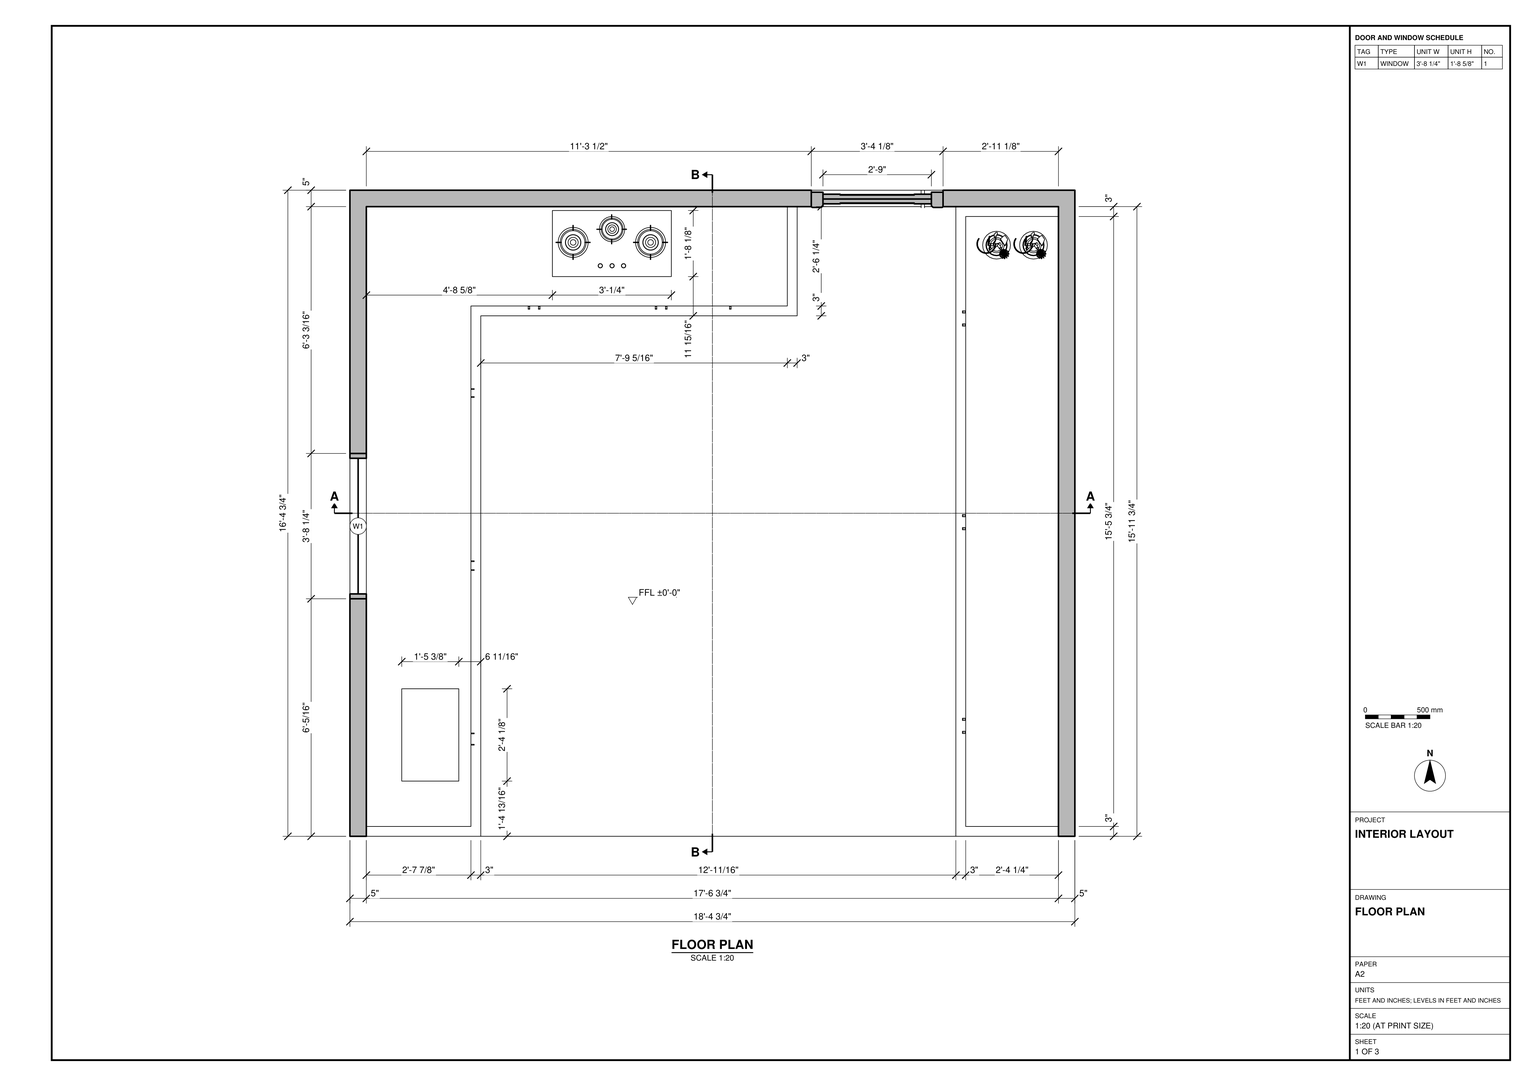
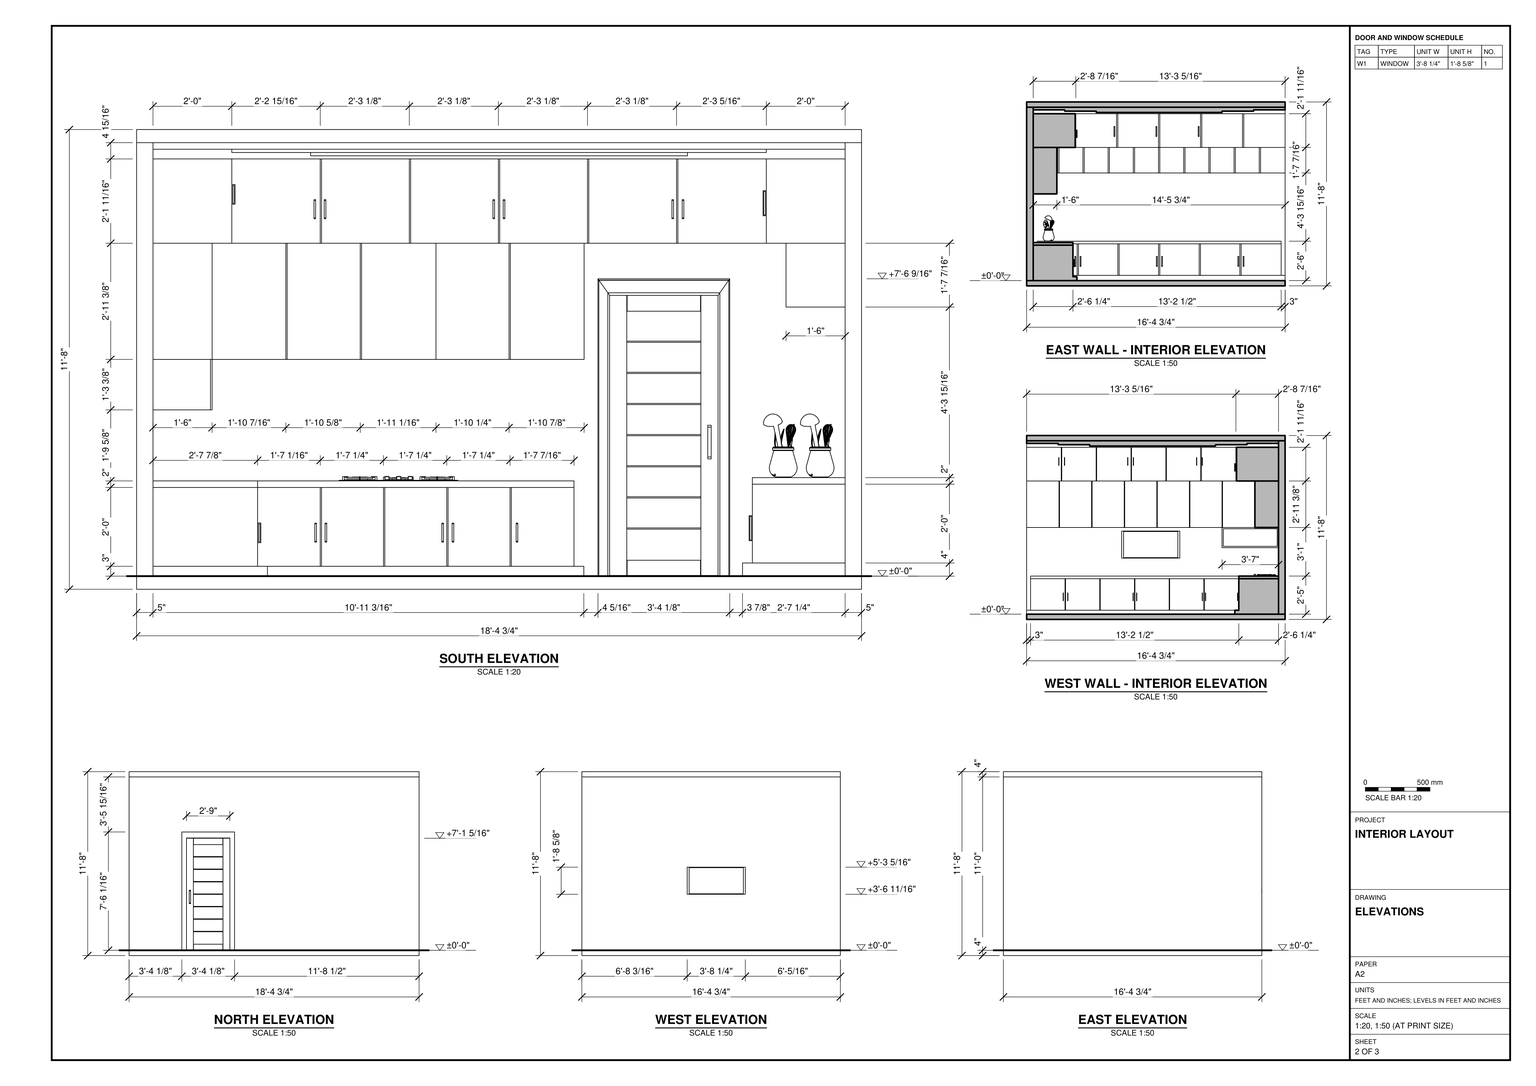
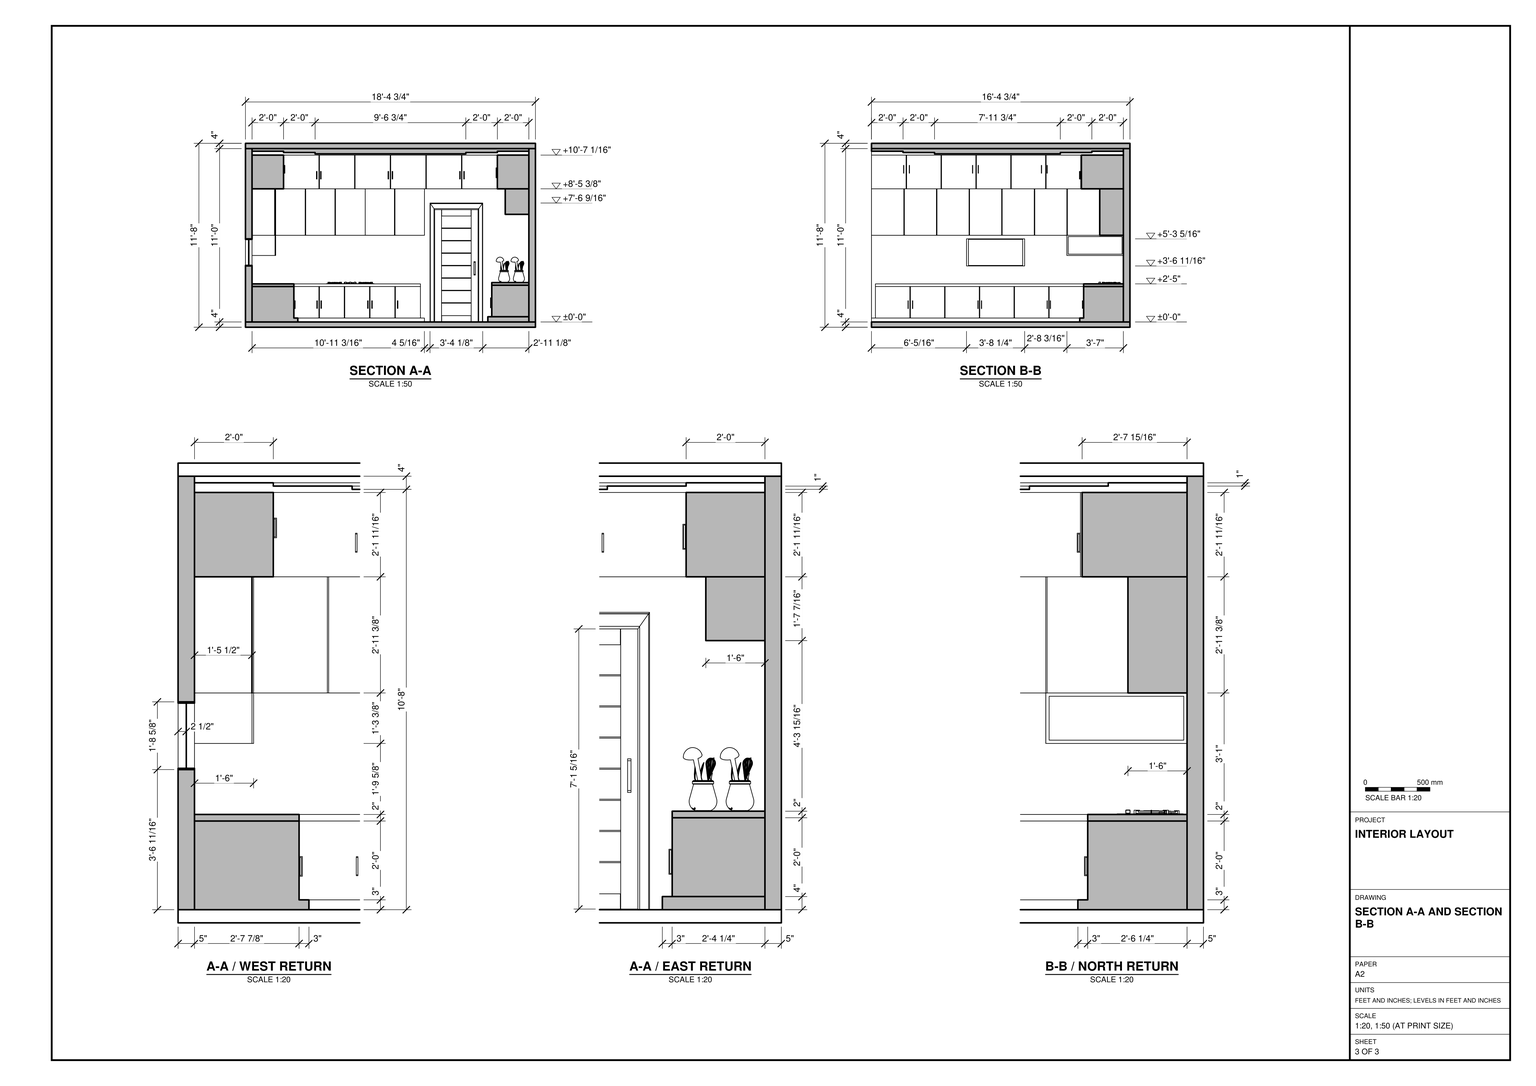
Build the kitchen in SketchUp using the plan, elevations and sections in task_files/diagram_01.pdf. Work in feet and inches. Set the finished floor at ±0'-0". The overall shell is 18'-4 3/4" wide from east to west, 16'-4 3/4" deep from north to south and 11'-8" high. Model the 5" walls on the north, east and west sides, leaving the south side open as drawn. Include the floor and ceiling slabs and the stepped ceiling detail shown in section.

Fit the framed window above the west worktop and the horizontally panelled door in the north wall. Run the west base cabinets around the northwest corner to form the cooktop counter, stopping short of the door. Include the rectangular inset near the open end of the west worktop. Place the separate straight cabinet run against the east wall. Use the return sections to set the counter depths, plinths and worktop thicknesses. Match the cabinet front divisions, handles and tiers of overhead storage to the elevations, including the cabinet row above the door.

Decor and loose items, including the cooktop and countertop utensil holders, may be any suitable library components. Keep shell elements and individual furniture or joinery pieces in separate groups or components, and use components for repeated parts. Save one SketchUp model as output_files/kitchen_interior_and_its_fitted_cabinetry.skp.

# SketchUp Ruby script. Lengths in inches.
U = 1.inch
M = Sketchup.active_model
def pt(a) = Geom::Point3d.new(a.map { |v| v * U })
def face(e, loops, mat)
  f = e.add_face(loops[0].map { |a| pt(a) })
  loops[1..].each { |l| e.add_face(l.map { |a| pt(a) }).erase! }
  f.material = f.back_material = mat if mat
  f
end
# faces: each face lists its corners as indices into pts; further lists are holes
def faces(e, pts, list, mat = nil) = list.each { |f| face(e, (f[0].is_a?(Array) ? f : [f]).map { |l| l.map { |i| pts[i] } }, mat) }
# xy, xz, yz: faces in a plane at the given z, y or x. An outline is a flat list of corners, or four numbers for a rectangle; further outlines are holes
def ring(l) = l.size == 4 ? [[l[0], l[1]], [l[2], l[1]], [l[2], l[3]], [l[0], l[3]]] : l.each_slice(2).to_a
def flat(e, list, mat, &to3) = list.each { |f| face(e, (f[0].is_a?(Array) ? f : [f]).map { |l| ring(l).map { |u, v| to3.(u, v) } }, mat) }
def xy(e, z, list, mat = nil) = flat(e, list, mat) { |x, y| [x, y, z] }
def xz(e, y, list, mat = nil) = flat(e, list, mat) { |x, z| [x, y, z] }
def yz(e, x, list, mat = nil) = flat(e, list, mat) { |y, z| [x, y, z] }
def lines(e, pts, list) = list.each { |a, b| e.add_line(pt(pts[a]), pt(pts[b])) }
# prism: a flat outline (further loops are holes) pulled along v
def prism(e, loops, v, mat = nil)
  f = face(e, loops, mat); d = Geom::Vector3d.new(v.map { |x| x * U })
  f.pushpull(f.normal.samedirection?(d) ? d.length : -d.length)
end
def box(e, o, s, mat = nil) = prism(e, [[o, [o[0] + s[0], o[1], o[2]], [o[0] + s[0], o[1] + s[1], o[2]], [o[0], o[1] + s[1], o[2]]]], [0, 0, s[2]], mat)
def at(x, y, z, deg = 0) = Geom::Transformation.translation(pt([x, y, z])) * Geom::Transformation.rotation(ORIGIN, Z_AXIS, deg.degrees)
def axes(o, x, y, z) = Geom::Transformation.new([*x, 0, *y, 0, *z, 0, *pt(o).to_a, 1])
def part(name) = M.definitions.add(name)
# library, detail: a bought-in or finely detailed component or shape, given as its bounding box
def library(name, o, s) = part(name).tap { |d| box(d.entities, o, s) }
def detail(e, o, s) = box(e.add_group.entities, o, s)
def put(e, d, t, mat = nil) = e.add_instance(d, t).tap { |i| i.material = mat if mat }
def group(e, t, mat = nil) = e.add_group.tap { |g| g.transformation = t; g.material = mat if mat }.entities
root = M.entities
M.materials.add("CROMO PERFIL METALICO").color = [144, 144, 144]
M.materials.add("Emissive").color = [255, 255, 255]
M.materials.add("MADEIRAS PORTAS MOD 4").color = [48, 37, 30]
M.materials.add("[Aluminum]").color = [179, 179, 179]
M.materials.add("[Carrera Marble]").color = [255, 255, 255]
M.materials.add("[Color D01]").color = [255, 242, 204]
M.materials.add("[Color E01]").color = [255, 255, 204]
M.materials.add("[Color F02]").color = [204, 255, 153]
M.materials.add("[Color M07]").color = [58, 58, 58]
M.materials.add("[Terrazzo Tile Accent]").color = [224, 221, 217]
M.materials.add("[Translucent Glass Gray]3").color = [128, 128, 128]
M.materials["[Translucent Glass Gray]3"].alpha = 0.3
M.materials.add("[Translucent Glass Sky Reflection]").color = [126, 138, 183]
M.materials["[Translucent Glass Sky Reflection]"].alpha = 0.52
M.materials.add("[Wood Cherry Original]").color = [152, 86, 42]
c1 = part("Group\#12")
xy(c1.entities,0,[[-0.79,16.82,0.71,16.85],[-0.79,16.85,0.71,23.5],[-0.79,23.5,0.71,23.53]],"CROMO PERFIL METALICO")
xy(c1.entities,0.39,[[-0.79,17.125,0.71,23.23]],"CROMO PERFIL METALICO")
xy(c1.entities,1.97,[[-0.79,16.73,0.71,17.125],[-0.79,23.23,0.71,23.62]],"CROMO PERFIL METALICO")
xz(c1.entities,16.73,[[-0.79,0.12,0.71,1.97]],"CROMO PERFIL METALICO")
xz(c1.entities,17.125,[[-0.79,0.39,0.71,1.97]],"CROMO PERFIL METALICO")
xz(c1.entities,23.23,[[-0.79,0.39,0.71,1.97]],"CROMO PERFIL METALICO")
xz(c1.entities,23.62,[[-0.79,0.09,0.71,0.12],[-0.79,0.12,0.71,1.97]],"CROMO PERFIL METALICO")
yz(c1.entities,-0.79,[[16.82,0,16.79,0.02,16.77,0.03,16.75,0.06,16.73,0.12,16.73,1.97,17.125,1.97,17.125,0.39,23.23,0.39,23.23,1.97,23.62,1.97,23.62,0.09,23.61,0.06,23.59,0.03,23.5625,0.02,23.53,0]],"CROMO PERFIL METALICO")
yz(c1.entities,0.71,[[16.82,0,23.53,0,23.5625,0.02,23.59,0.03,23.61,0.06,23.62,0.09,23.62,1.97,23.23,1.97,23.23,0.39,17.125,0.39,17.125,1.97,16.73,1.97,16.73,0.12,16.75,0.06,16.77,0.03,16.79,0.02]],"CROMO PERFIL METALICO")
p = [[-0.79,16.75,0.06],[-0.79,16.77,0.03],[0.71,16.77,0.03],[0.71,16.75,0.06],[-0.79,16.79,0.02],[0.71,16.79,0.02],
  [-0.79,16.82,0],[0.71,16.82,0],[-0.79,23.53,0],[-0.79,23.5625,0.02],[0.71,23.5625,0.02],[0.71,23.53,0],
  [-0.79,23.59,0.03],[0.71,23.59,0.03],[-0.79,23.61,0.06],[0.71,23.61,0.06],[-0.79,16.73,0.12],[-0.79,16.74,0.09],
  [0.71,16.74,0.09],[0.71,16.73,0.12],[-0.79,23.62,0.09],[0.71,23.62,0.09]]
faces(c1.entities,p,[[0,1,2,3],[1,4,5,2],[4,6,7,5],[8,9,10,11],[9,12,13,10],[12,14,15,13],[16,17,18,19],[17,0,3,18],
  [14,20,21,15]],"CROMO PERFIL METALICO")
c2 = part("Framed door panel")
xy(c2.entities,0.21,[[0,0,2.36,0,2.36,7.48,2.17,7.48,2.17,7.64,2.36,7.64,2.36,39.61,2.17,39.61,2.17,39.76,2.36,39.76,2.36,47.24,0,47.24]],"MADEIRAS PORTAS MOD 4")
xy(c2.entities,5.12,[[1.97,7.48,2.17,7.48,2.17,7.64,2.36,7.64,2.36,39.61,2.17,39.61,2.17,39.76,1.97,39.76]],"MADEIRAS PORTAS MOD 4")
xy(c2.entities,15.16,[[1.57,7.48,1.97,39.76]],"MADEIRAS PORTAS MOD 4")
xy(c2.entities,15.55,[[1.57,7.48,1.97,39.76]],"MADEIRAS PORTAS MOD 4")
xy(c2.entities,25.2,[[1.57,7.48,1.97,39.76]],"MADEIRAS PORTAS MOD 4")
xy(c2.entities,25.59,[[1.57,7.48,1.97,39.76]],"MADEIRAS PORTAS MOD 4")
xy(c2.entities,35.24,[[1.57,7.48,1.97,39.76]],"MADEIRAS PORTAS MOD 4")
xy(c2.entities,35.63,[[1.57,7.48,1.97,39.76]],"MADEIRAS PORTAS MOD 4")
xy(c2.entities,45.28,[[1.57,7.48,1.97,39.76]],"MADEIRAS PORTAS MOD 4")
xy(c2.entities,45.67,[[1.57,7.48,1.97,39.76]],"MADEIRAS PORTAS MOD 4")
xy(c2.entities,55.31,[[1.57,7.48,1.97,39.76]],"MADEIRAS PORTAS MOD 4")
xy(c2.entities,55.71,[[1.57,7.48,1.97,39.76]],"MADEIRAS PORTAS MOD 4")
xy(c2.entities,65.35,[[1.57,7.48,1.97,39.76]],"MADEIRAS PORTAS MOD 4")
xy(c2.entities,65.75,[[1.57,7.48,1.97,39.76]],"MADEIRAS PORTAS MOD 4")
xy(c2.entities,75.39,[[1.57,7.48,1.97,39.76]],"MADEIRAS PORTAS MOD 4")
xy(c2.entities,75.79,[[1.57,7.48,1.97,39.76]],"MADEIRAS PORTAS MOD 4")
xy(c2.entities,85.43,[[1.97,7.48,1.97,39.76,2.17,39.76,2.17,39.61,2.36,39.61,2.36,7.64,2.17,7.64,2.17,7.48]],"MADEIRAS PORTAS MOD 4")
xy(c2.entities,90.55,[[0,0,2.36,0,2.36,7.48,2.17,7.48,2.17,7.64,2.36,7.64,2.36,39.61,2.17,39.61,2.17,39.76,2.36,39.76,2.36,47.24,0,47.24]],"MADEIRAS PORTAS MOD 4")
xz(c2.entities,0,[[0,0.21,2.36,90.55]],"MADEIRAS PORTAS MOD 4")
xz(c2.entities,7.48,[[2.17,0.21,2.36,5.12],[1.97,5.12,2.36,15.16],[1.57,15.16,1.57,15.55,1.97,15.55,1.97,25.2,2.36,25.2,2.36,15.16],[1.57,25.2,1.57,25.59,1.97,25.59,1.97,35.24,2.36,35.24,2.36,25.2],[1.57,35.24,1.57,35.63,1.97,35.63,1.97,45.28,2.36,45.28,2.36,35.24],
  [1.57,45.28,1.57,45.67,1.97,45.67,1.97,55.31,2.36,55.31,2.36,45.28],[1.57,55.31,1.57,55.71,1.97,55.71,1.97,65.35,2.36,65.35,2.36,55.31],[1.57,65.35,1.57,65.75,1.97,65.75,1.97,75.39,2.36,75.39,2.36,65.35],[1.57,75.39,1.57,75.79,1.97,75.79,1.97,85.43,2.36,85.43,2.36,75.39],[2.17,85.43,2.36,90.55]],"MADEIRAS PORTAS MOD 4")
xz(c2.entities,7.64,[[2.17,0.21,2.36,5.12],[2.17,85.43,2.36,90.55]],"MADEIRAS PORTAS MOD 4")
xz(c2.entities,39.61,[[2.17,0.21,2.36,5.12],[2.17,85.43,2.36,90.55]],"MADEIRAS PORTAS MOD 4")
xz(c2.entities,39.76,[[2.17,0.21,2.36,5.12],[1.97,5.12,2.36,15.16],[1.57,15.16,2.36,15.16,2.36,25.2,1.97,25.2,1.97,15.55,1.57,15.55],[1.57,25.2,2.36,25.2,2.36,35.24,1.97,35.24,1.97,25.59,1.57,25.59],[1.57,35.24,2.36,35.24,2.36,45.28,1.97,45.28,1.97,35.63,1.57,35.63],
  [1.57,45.28,2.36,45.28,2.36,55.31,1.97,55.31,1.97,45.67,1.57,45.67],[1.57,55.31,2.36,55.31,2.36,65.35,1.97,65.35,1.97,55.71,1.57,55.71],[1.57,65.35,2.36,65.35,2.36,75.39,1.97,75.39,1.97,65.75,1.57,65.75],[1.57,75.39,2.36,75.39,2.36,85.43,1.97,85.43,1.97,75.79,1.57,75.79],[2.17,85.43,2.36,90.55]],"MADEIRAS PORTAS MOD 4")
xz(c2.entities,47.24,[[0,0.21,2.36,90.55]],"MADEIRAS PORTAS MOD 4")
yz(c2.entities,0,[[0,0.21,47.24,90.55]],"MADEIRAS PORTAS MOD 4")
yz(c2.entities,1.57,[[7.48,15.16,39.76,15.55],[7.48,25.2,39.76,25.59],[7.48,35.24,39.76,35.63],[7.48,45.28,39.76,45.67],[7.48,55.31,39.76,55.71],
  [7.48,65.35,39.76,65.75],[7.48,75.39,39.76,75.79]],"MADEIRAS PORTAS MOD 4")
yz(c2.entities,1.97,[[7.48,5.12,39.76,15.16],[7.48,15.55,39.76,25.2],[7.48,25.59,39.76,35.24],[7.48,35.63,39.76,45.28],[7.48,45.67,39.76,55.31],
  [7.48,55.71,39.76,65.35],[7.48,65.75,39.76,75.39],[7.48,75.79,39.76,85.43]],"MADEIRAS PORTAS MOD 4")
yz(c2.entities,2.17,[[7.48,0.21,7.64,5.12],[39.61,0.21,39.76,5.12],[7.48,85.43,7.64,90.55],[39.61,85.43,39.76,90.55]],"MADEIRAS PORTAS MOD 4")
yz(c2.entities,2.36,[[0,0.21,7.48,90.55],[7.64,0.21,39.61,5.12],[39.76,0.21,47.24,90.55],[7.64,85.43,39.61,90.55]],"MADEIRAS PORTAS MOD 4")
put(c2.entities,c1,axes([4.33,43.46,11.46],[0,-1,0],[0,0,1.575],[-1,0,0]))
c3 = part("Framed door panel \#1")
xy(c3.entities,0.21,[[0,0,2.36,0,2.36,7.48,2.17,7.48,2.17,7.64,2.36,7.64,2.36,39.61,2.17,39.61,2.17,39.76,2.36,39.76,2.36,47.24,0,47.24]],"MADEIRAS PORTAS MOD 4")
xy(c3.entities,5.12,[[1.97,7.48,2.17,7.48,2.17,7.64,2.36,7.64,2.36,39.61,2.17,39.61,2.17,39.76,1.97,39.76]],"MADEIRAS PORTAS MOD 4")
xy(c3.entities,15.16,[[1.57,7.48,1.97,39.76]],"MADEIRAS PORTAS MOD 4")
xy(c3.entities,15.55,[[1.57,7.48,1.97,39.76]],"MADEIRAS PORTAS MOD 4")
xy(c3.entities,25.2,[[1.57,7.48,1.97,39.76]],"MADEIRAS PORTAS MOD 4")
xy(c3.entities,25.59,[[1.57,7.48,1.97,39.76]],"MADEIRAS PORTAS MOD 4")
xy(c3.entities,35.24,[[1.57,7.48,1.97,39.76]],"MADEIRAS PORTAS MOD 4")
xy(c3.entities,35.63,[[1.57,7.48,1.97,39.76]],"MADEIRAS PORTAS MOD 4")
xy(c3.entities,45.28,[[1.57,7.48,1.97,39.76]],"MADEIRAS PORTAS MOD 4")
xy(c3.entities,45.67,[[1.57,7.48,1.97,39.76]],"MADEIRAS PORTAS MOD 4")
xy(c3.entities,55.31,[[1.57,7.48,1.97,39.76]],"MADEIRAS PORTAS MOD 4")
xy(c3.entities,55.71,[[1.57,7.48,1.97,39.76]],"MADEIRAS PORTAS MOD 4")
xy(c3.entities,65.35,[[1.57,7.48,1.97,39.76]],"MADEIRAS PORTAS MOD 4")
xy(c3.entities,65.75,[[1.57,7.48,1.97,39.76]],"MADEIRAS PORTAS MOD 4")
xy(c3.entities,75.39,[[1.57,7.48,1.97,39.76]],"MADEIRAS PORTAS MOD 4")
xy(c3.entities,75.79,[[1.57,7.48,1.97,39.76]],"MADEIRAS PORTAS MOD 4")
xy(c3.entities,85.43,[[1.97,7.48,1.97,39.76,2.17,39.76,2.17,39.61,2.36,39.61,2.36,7.64,2.17,7.64,2.17,7.48]],"MADEIRAS PORTAS MOD 4")
xy(c3.entities,90.55,[[0,0,2.36,0,2.36,7.48,2.17,7.48,2.17,7.64,2.36,7.64,2.36,39.61,2.17,39.61,2.17,39.76,2.36,39.76,2.36,47.24,0,47.24]],"MADEIRAS PORTAS MOD 4")
xz(c3.entities,0,[[0,0.21,2.36,90.55]],"MADEIRAS PORTAS MOD 4")
xz(c3.entities,7.48,[[2.17,0.21,2.36,5.12],[1.97,5.12,2.36,15.16],[1.57,15.16,1.57,15.55,1.97,15.55,1.97,25.2,2.36,25.2,2.36,15.16],[1.57,25.2,1.57,25.59,1.97,25.59,1.97,35.24,2.36,35.24,2.36,25.2],[1.57,35.24,1.57,35.63,1.97,35.63,1.97,45.28,2.36,45.28,2.36,35.24],
  [1.57,45.28,1.57,45.67,1.97,45.67,1.97,55.31,2.36,55.31,2.36,45.28],[1.57,55.31,1.57,55.71,1.97,55.71,1.97,65.35,2.36,65.35,2.36,55.31],[1.57,65.35,1.57,65.75,1.97,65.75,1.97,75.39,2.36,75.39,2.36,65.35],[1.57,75.39,1.57,75.79,1.97,75.79,1.97,85.43,2.36,85.43,2.36,75.39],[2.17,85.43,2.36,90.55]],"MADEIRAS PORTAS MOD 4")
xz(c3.entities,7.64,[[2.17,0.21,2.36,5.12],[2.17,85.43,2.36,90.55]],"MADEIRAS PORTAS MOD 4")
xz(c3.entities,39.61,[[2.17,0.21,2.36,5.12],[2.17,85.43,2.36,90.55]],"MADEIRAS PORTAS MOD 4")
xz(c3.entities,39.76,[[2.17,0.21,2.36,5.12],[1.97,5.12,2.36,15.16],[1.57,15.16,2.36,15.16,2.36,25.2,1.97,25.2,1.97,15.55,1.57,15.55],[1.57,25.2,2.36,25.2,2.36,35.24,1.97,35.24,1.97,25.59,1.57,25.59],[1.57,35.24,2.36,35.24,2.36,45.28,1.97,45.28,1.97,35.63,1.57,35.63],
  [1.57,45.28,2.36,45.28,2.36,55.31,1.97,55.31,1.97,45.67,1.57,45.67],[1.57,55.31,2.36,55.31,2.36,65.35,1.97,65.35,1.97,55.71,1.57,55.71],[1.57,65.35,2.36,65.35,2.36,75.39,1.97,75.39,1.97,65.75,1.57,65.75],[1.57,75.39,2.36,75.39,2.36,85.43,1.97,85.43,1.97,75.79,1.57,75.79],[2.17,85.43,2.36,90.55]],"MADEIRAS PORTAS MOD 4")
xz(c3.entities,47.24,[[0,0.21,2.36,90.55]],"MADEIRAS PORTAS MOD 4")
yz(c3.entities,0,[[0,0.21,47.24,90.55]],"MADEIRAS PORTAS MOD 4")
yz(c3.entities,1.57,[[7.48,15.16,39.76,15.55],[7.48,25.2,39.76,25.59],[7.48,35.24,39.76,35.63],[7.48,45.28,39.76,45.67],[7.48,55.31,39.76,55.71],
  [7.48,65.35,39.76,65.75],[7.48,75.39,39.76,75.79]],"MADEIRAS PORTAS MOD 4")
yz(c3.entities,1.97,[[7.48,5.12,39.76,15.16],[7.48,15.55,39.76,25.2],[7.48,25.59,39.76,35.24],[7.48,35.63,39.76,45.28],[7.48,45.67,39.76,55.31],
  [7.48,55.71,39.76,65.35],[7.48,65.75,39.76,75.39],[7.48,75.79,39.76,85.43]],"MADEIRAS PORTAS MOD 4")
yz(c3.entities,2.17,[[7.48,0.21,7.64,5.12],[39.61,0.21,39.76,5.12],[7.48,85.43,7.64,90.55],[39.61,85.43,39.76,90.55]],"MADEIRAS PORTAS MOD 4")
yz(c3.entities,2.36,[[0,0.21,7.48,90.55],[7.64,0.21,39.61,5.12],[39.76,0.21,47.24,90.55],[7.64,85.43,39.61,90.55]],"MADEIRAS PORTAS MOD 4")
put(c3.entities,c1,axes([4.33,3.7,11.46],[0,-1,0],[0,0,1.575],[-1,0,0]))
c4 = part("Agrupar\#1")
xy(c4.entities,0,[[-0.94,0,-1.34,0.39,-1.34,7.48,3.78,7.48,3.78,0.79,2.99,0],[52.125,0,51.34,0.79,51.34,7.48,56.46,7.48,56.46,0.39,56.0625,0]],"MADEIRAS PORTAS MOD 4")
xy(c4.entities,86.77,[[3.78,0.79,51.34,7.09],[3.78,7.09,51.34,7.48]],"MADEIRAS PORTAS MOD 4")
xy(c4.entities,91.89,[[-1.34,0.39,56.46,7.48]],"MADEIRAS PORTAS MOD 4")
xz(c4.entities,0,[[-0.94,0,2.99,0,2.99,87.56,-0.94,91.5],[52.125,0,56.0625,0,56.0625,91.5,52.125,87.56],[2.99,87.56,52.125,87.56,56.0625,91.5,-0.94,91.5]],"MADEIRAS PORTAS MOD 4")
xz(c4.entities,7.48,[[-1.34,0,3.78,0,3.78,86.77,51.34,86.77,51.34,0,56.46,0,56.46,91.89,-1.34,91.89]],"MADEIRAS PORTAS MOD 4")
yz(c4.entities,-1.34,[[0.39,0,7.48,91.89]],"MADEIRAS PORTAS MOD 4")
yz(c4.entities,3.78,[[0.79,0,7.48,86.77]],"MADEIRAS PORTAS MOD 4")
yz(c4.entities,51.34,[[0.79,0,7.09,86.77],[7.09,0,7.48,86.77]],"MADEIRAS PORTAS MOD 4")
yz(c4.entities,56.46,[[0.39,0,7.48,91.89]],"MADEIRAS PORTAS MOD 4")
p = [[-1.34,0.39,0],[-0.94,0,0],[-0.94,0,91.5],[-1.34,0.39,91.89],[3.78,0.79,86.77],[2.99,0,87.56],
  [2.99,0,0],[3.78,0.79,0],[51.34,0.79,0],[52.125,0,0],[52.125,0,87.56],[51.34,0.79,86.77],
  [56.46,0.39,91.89],[56.0625,0,91.5],[56.0625,0,0],[56.46,0.39,0]]
faces(c4.entities,p,[[0,1,2,3],[4,5,6,7],[8,9,10,11],[12,13,14,15],[11,10,5,4],[3,2,13,12]],"MADEIRAS PORTAS MOD 4")
c5 = part("建立群組\#94")
put(c5.entities,c2,axes([2.85,32.65,-0.17],[-0.65909,0,0],[0,-0.62402,0],[0,0,0.82113]),"MADEIRAS PORTAS MOD 4")
put(c5.entities,c3,axes([2.85,3.17,0],[0.65909,0,0],[0,0.62402,0],[0,0,0.82113]),"MADEIRAS PORTAS MOD 4")
put(c5.entities,c4,axes([5.58,0.83,0],[0,0.61989,0],[-0.65909,0,0],[0,0,0.8569]),"MADEIRAS PORTAS MOD 4")
c6 = part("元件\#5")
put(c6.entities,c5,axes([0.98,0,0],[-0.94122,0,0],[0,1,0],[0,0,1.15]))
c7 = part("WINDOW (1)")
xy(c7.entities,0,[[0,0,59.06,1.97]],"[Color M07]")
xy(c7.entities,1.97,[[1.97,0,57.09,0.98],[1.97,0.98,57.09,1.97]],"[Color M07]")
xy(c7.entities,104.33,[[1.97,0,57.09,0.98],[1.97,0.98,57.09,1.97]],"[Color M07]")
xy(c7.entities,106.3,[[0,0,59.06,1.97]],"[Color M07]")
xz(c7.entities,0,[[[0,0,59.06,106.3],[1.97,1.97,57.09,104.33]]],"[Color M07]")
xz(c7.entities,0.98,[[1.97,1.97,57.09,104.33]],"[Translucent Glass Gray]3")
xz(c7.entities,1.97,[[[0,0,59.06,106.3],[1.97,1.97,57.09,104.33]]],"[Color M07]")
yz(c7.entities,0,[[0,0,1.97,106.3]],"[Color M07]")
yz(c7.entities,1.97,[[0,1.97,0.98,104.33],[0.98,1.97,1.97,104.33]],"[Color M07]")
yz(c7.entities,57.09,[[0,1.97,0.98,104.33],[0.98,1.97,1.97,104.33]],"[Color M07]")
yz(c7.entities,59.06,[[0,0,1.97,106.3]],"[Color M07]")
c8 = library("utensils3",[0.34,2.72,-0.74],[8.53,6.44,13.22])
c9 = library("Bosch Stove",[0,0,0],[36.22,20.12,1.38])
c10 = part("Group\#21")
prism(c10.entities,[[[0,0,6],[0,0,0],[1,0,0],[1,0,6]],[[0.28,0,5.72],[0.72,0,5.72],[0.72,0,0.28],[0.28,0,0.28]]],[0,0.25,0])
c11 = part("Group\#22")
prism(c11.entities,[[[0.5,1,0],[0.5,1,5.8125],[0.5,0,5.8125],[0.5,0,0]],[[0.5,0.74,0.26],[0.5,0.26,0.26],[0.5,0.26,5.55],[0.5,0.74,5.55]]],[-0.5,0,0])
c12 = part("Group\#23")
prism(c12.entities,[[[1,0,0],[1,0,7.625],[0,0,7.625],[0,0,0]],[[0.76,0,7.38],[0.76,0,0.24],[0.24,0,0.24],[0.24,0,7.38]]],[0,0.6875,0])
xy(root,32,[[187.51,3,215.75,188.75]])
xy(root,34,[[187.51,3,215.75,188.75]],"[Carrera Marble]")
xz(root,3,[[187.51,32,215.75,34]])
xz(root,188.75,[[187.51,32,215.75,34]])
yz(root,22.5,[[49.84,70,74.66,105.37],[74.66,70,99.09,105.37]],"[Translucent Glass Sky Reflection]")
yz(root,187.51,[[3,32,188.75,34]])
yz(root,215.75,[[3,32,188.75,34]])
p = [[23,191.75,54.625],[22.5,148.73,54.625],[22.5,148.73,70],[23,191.75,70],[91.16,173.75,105.37],[91.16,173.75,70],
  [68.51,174.25,70],[68.51,174.25,105.37]]
faces(root,p,[[0,1,2,3],[4,5,6,7]],"[Translucent Glass Sky Reflection]")
put(root,c6,axes([180.61,195.77,4],[0,1,0],[-1.12001,0,0],[0,0,1]))
put(root,c7,axes([0,72.34,46.67],[0,0.7493,0],[2.54,0,0],[0,0,0.19403]))
put(root,c8,axes([201.03,170.87,35.31],[1.5,0,0],[0,1.5,0],[0,0,1.5]))
put(root,c8,axes([189.78,170.87,35.31],[1.5,0,0],[0,1.5,0],[0,0,1.5]))
put(root,c9,at(61.65,170.45,33))
g1 = group(root,at(0,24,0),"[Terrazzo Tile Accent]")
box(g1,[0,-24,0],[220.75,196.75,4])
g2 = group(root,at(0,0,4),"[Color D01]")
xy(g2,0,[[140.49,191.75,180.61,196.75]])
xy(g2,42.67,[[0,72.34,5,116.59]])
xy(g2,63.29,[[0,72.34,5,116.59]])
xy(g2,90.08,[[140.49,191.75,180.61,196.75]])
xy(g2,132,[[0,0,5,0,5,191.75,215.75,191.75,215.75,0,220.75,0,220.75,196.75,0,196.75]])
xz(g2,0,[[0,0,5,132],[215.75,0,220.75,132]])
xz(g2,72.34,[[0,42.67,5,63.29]])
xz(g2,116.59,[[0,42.67,5,63.29]])
xz(g2,191.75,[[5,0,140.49,0,140.49,90.08,180.61,90.08,180.61,0,215.75,0,215.75,132,5,132]])
xz(g2,196.75,[[0,0,0,132,220.75,132,220.75,0,180.61,0,180.61,90.08,140.49,90.08,140.49,0]])
yz(g2,0,[[[0,0,196.75,132],[72.34,42.67,116.59,63.29]]])
yz(g2,5,[[[0,0,191.75,132],[72.34,42.67,116.59,63.29]]])
yz(g2,140.49,[[191.75,0,196.75,90.08]])
yz(g2,180.61,[[191.75,0,196.75,90.08]])
yz(g2,215.75,[[0,0,191.75,132]])
yz(g2,220.75,[[0,0,196.75,132]])
p = [[215.75,0,0],[5,0,0]]
lines(g2,p,[[0,1]])
g3 = group(root,at(191.75,0,105.37),"[Color F02]")
prism(g3,[[[24,191.75,0],[24,0,0],[0,0,0],[0,31.46,0],[0.5,31.46,0],[0.5,32.46,0],[0,32.46,0],[0,63.42,0],[0.5,63.42,0],[0.5,64.42,0],[0,64.42,0],[0,95.375,0],[0.5,95.375,0],[0.5,96.375,0],[0,96.375,0],[0,127.33,0],[0.5,127.33,0],[0.5,128.33,0],[0,128.33,0],[0,159.29,0],[0.5,159.29,0],[0.5,160.29,0],[0,160.29,0],[0,191.75,0]]],[0,0,25.68])
g4 = group(root,at(197.75,0,85.94),"[Color E01]")
prism(g4,[[[18,191.75,0],[18,0,0],[0,0,0],[0,18.68,0],[0.5,18.68,0],[0.5,19.68,0],[0,19.68,0],[0,37.85,0],[0.5,37.85,0],[0.5,38.85,0],[0,38.85,0],[0,57.03,0],[0.5,57.03,0],[0.5,58.03,0],[0,58.03,0],[0,76.2,0],[0.5,76.2,0],[0.5,77.2,0],[0,77.2,0],[0,95.375,0],[0.5,95.375,0],[0.5,96.375,0],[0,96.375,0],[0,114.55,0],[0.5,114.55,0],[0.5,115.55,0],[0,115.55,0],[0,133.73,0],[0.5,133.73,0],[0.5,134.73,0],[0,134.73,0],[0,152.9,0],[0.5,152.9,0],[0.5,153.9,0],[0,153.9,0],[0,172.08,0],[0.5,172.08,0],[0.5,173.08,0],[0,173.08,0],[0,191.75,0]]],[0,0,19.43])
g5 = group(root,at(184.51,0,4),"[Carrera Marble]")
box(g5,[0,0,0],[31.24,191.75,4])
g6 = group(root,at(5,159.29,105.37),"[Color F02]")
prism(g6,[[[0,32.46,0],[186.75,32.46,0],[186.75,0,0],[159.83,0,0],[159.83,0.5,0],[159.43,0.5,0],[159.43,0,0],[132.7,0,0],[132.7,0.5,0],[132.3,0.5,0],[132.3,0,0],[105.58,0,0],[105.58,0.5,0],[105.18,0.5,0],[105.18,0,0],[78.45,0,0],[78.45,0.5,0],[78.05,0.5,0],[78.05,0,0],[51.32,0,0],[51.32,0.5,0],[50.92,0.5,0],[50.92,0,0],[24,0,0],[0,0,0]]],[0,0,25.68])
g7 = group(root,at(5,0,105.37),"[Color F02]")
prism(g7,[[[0,0,0],[0,159.29,0],[24,159.29,0],[24,132.94,0],[23.5,132.94,0],[23.5,132.54,0],[24,132.54,0],[24,106.39,0],[23.5,106.39,0],[23.5,105.99,0],[24,105.99,0],[24,79.85,0],[23.5,79.85,0],[23.5,79.45,0],[24,79.45,0],[24,53.3,0],[23.5,53.3,0],[23.5,52.9,0],[24,52.9,0],[24,26.75,0],[23.5,26.75,0],[23.5,26.35,0],[24,26.35,0],[24,0,0]]],[0,0,25.68])
g8 = group(root,at(5,0,70),"[Color E01]")
xy(g8,0,[[0,0,0,49.84,17.5,49.84,17.5,49.44,18,49.44,18,25.02,17.5,25.02,17.5,24.62,18,24.62,18,0],[0,74.26,17.5,74.66],[0,99.09,0,191.75,18,191.75,18,149.13,17.5,149.13,17.5,148.73,18,148.73,18,124.31,17.5,124.31,17.5,123.91,18,123.91,18,99.49,17.5,99.49,17.5,99.09],[18,173.75,18,191.75,63.51,191.75,63.51,174.25,63.11,174.25,63.11,173.75,40.85,173.75,40.85,174.25,40.45,174.25,40.45,173.75],[86.16,173.75,86.16,174.25,85.76,174.25,85.76,191.75,131.27,191.75,131.27,173.75,108.8125,173.75,108.8125,174.25,108.41,174.25,108.41,173.75]])
xy(g8,35.37,[[0,0,18,0,18,24.62,17.5,24.62,17.5,25.02,18,25.02,18,49.44,17.5,49.44,17.5,49.84,0,49.84],[0,74.26,17.5,74.66],[0,99.09,17.5,99.09,17.5,99.49,18,99.49,18,123.91,17.5,123.91,17.5,124.31,18,124.31,18,148.73,17.5,148.73,17.5,149.13,18,149.13,18,191.75,0,191.75],[18,173.75,40.45,173.75,40.45,174.25,40.85,174.25,40.85,173.75,63.11,173.75,63.11,174.25,63.51,174.25,63.51,191.75,18,191.75],[86.16,173.75,108.41,173.75,108.41,174.25,108.8125,174.25,108.8125,173.75,131.27,173.75,131.27,191.75,85.76,191.75,85.76,174.25,86.16,174.25]])
xz(g8,0,[[0,0,18,35.37]])
xz(g8,24.62,[[17.5,0,18,35.37]])
xz(g8,25.02,[[17.5,0,18,35.37]])
xz(g8,49.44,[[17.5,0,18,35.37]])
xz(g8,49.84,[[0,0,17.5,35.37]])
xz(g8,74.26,[[0,0,17.5,35.37]])
xz(g8,74.66,[[0,0,17.5,35.37]])
xz(g8,99.09,[[0,0,17.5,35.37]])
xz(g8,99.49,[[17.5,0,18,35.37]])
xz(g8,123.91,[[17.5,0,18,35.37]])
xz(g8,124.31,[[17.5,0,18,35.37]])
xz(g8,148.73,[[17.5,0,18,35.37]])
xz(g8,149.13,[[17.5,0,18,35.37]])
xz(g8,173.75,[[18,0,40.45,35.37],[40.85,0,63.11,35.37],[86.16,0,108.41,35.37],[108.8125,0,131.27,35.37]])
xz(g8,174.25,[[40.45,0,40.85,35.37],[63.11,0,63.51,35.37],[85.76,0,86.16,35.37],[108.41,0,108.8125,35.37]])
xz(g8,191.75,[[18,0,63.51,35.37],[63.51,0,85.76,35.37],[85.76,0,131.27,35.37]])
yz(g8,0,[[0,0,49.84,35.37],[49.84,0,74.26,35.37],[74.26,0,74.66,35.37],[74.66,0,99.09,35.37],[99.09,0,191.75,35.37]])
yz(g8,17.5,[[24.62,0,25.02,35.37],[49.44,0,49.84,35.37],[74.26,0,74.66,35.37],[99.09,0,99.49,35.37],[123.91,0,124.31,35.37],
  [148.73,0,149.13,35.37]])
yz(g8,18,[[0,0,24.62,35.37],[25.02,0,49.44,35.37],[99.49,0,123.91,35.37],[124.31,0,148.73,35.37],[149.13,0,173.75,35.37]])
yz(g8,40.45,[[173.75,0,174.25,35.37]])
yz(g8,40.85,[[173.75,0,174.25,35.37]])
yz(g8,63.11,[[173.75,0,174.25,35.37]])
yz(g8,63.51,[[174.25,0,191.75,35.37]])
yz(g8,85.76,[[174.25,0,191.75,35.37]])
yz(g8,86.16,[[173.75,0,174.25,35.37]])
yz(g8,108.41,[[173.75,0,174.25,35.37]])
yz(g8,108.8125,[[173.75,0,174.25,35.37]])
yz(g8,131.27,[[173.75,0,191.75,35.37]])
g9 = group(root,at(5,0,4),"[Color F02]")
xy(g9,0,[[0,0,0,191.75,131.1875,191.75,131.1875,158.5,34.85,158.5,34.85,0]])
xy(g9,3,[[0,0,34.85,0,34.85,158.5,131.1875,158.5,131.1875,191.75,128.1875,191.75,128.1875,161.5,109.12,161.5,109.12,162,108.72,162,108.72,161.5,89.85,161.5,89.85,162,89.45,162,89.45,161.5,70.58,161.5,70.58,162,70.18,162,70.18,161.5,51.31,161.5,51.31,162,50.91,162,50.91,161.5,31.85,161.5,31.85,135.28,31.35,135.28,31.35,134.88,31.85,134.88,31.85,108.87,31.35,108.87,31.35,108.47,31.85,108.47,31.85,82.45,31.35,82.45,31.35,82.05,31.85,82.05,31.85,56.03,31.35,56.03,31.35,55.63,31.85,55.63,31.85,29.62,31.35,29.62,31.35,29.22,31.85,29.22,31.85,3,0,3]],"[Carrera Marble]")
xy(g9,27,[[0,3,31.85,3,31.85,29.22,31.35,29.22,31.35,29.62,31.85,29.62,31.85,55.63,31.35,55.63,31.35,56.03,31.85,56.03,31.85,82.05,31.35,82.05,31.35,82.45,31.85,82.45,31.85,108.47,31.35,108.47,31.35,108.87,31.85,108.87,31.85,134.88,31.35,134.88,31.35,135.28,31.85,135.28,31.85,161.5,50.91,161.5,50.91,162,51.31,162,51.31,161.5,70.18,161.5,70.18,162,70.58,162,70.58,161.5,89.45,161.5,89.45,162,89.85,162,89.85,161.5,108.72,161.5,108.72,162,109.12,162,109.12,161.5,128.1875,161.5,128.1875,191.75,0,191.75]],"[Carrera Marble]")
xz(g9,0,[[0,0,34.85,3]],"[Carrera Marble]")
xz(g9,3,[[0,3,31.85,27]])
xz(g9,29.22,[[31.35,3,31.85,27]])
xz(g9,29.62,[[31.35,3,31.85,27]])
xz(g9,55.63,[[31.35,3,31.85,27]])
xz(g9,56.03,[[31.35,3,31.85,27]])
xz(g9,82.05,[[31.35,3,31.85,27]])
xz(g9,82.45,[[31.35,3,31.85,27]])
xz(g9,108.47,[[31.35,3,31.85,27]])
xz(g9,108.87,[[31.35,3,31.85,27]])
xz(g9,134.88,[[31.35,3,31.85,27]])
xz(g9,135.28,[[31.35,3,31.85,27]])
xz(g9,158.5,[[34.85,0,131.1875,3]],"[Carrera Marble]")
xz(g9,161.5,[[31.85,3,50.91,27],[51.31,3,70.18,27],[70.58,3,89.45,27],[89.85,3,108.72,27],[109.12,3,128.1875,27]])
xz(g9,162,[[50.91,3,51.31,27],[70.18,3,70.58,27],[89.45,3,89.85,27],[108.72,3,109.12,27]])
xz(g9,191.75,[[0,0,0,27,128.1875,27,128.1875,3,131.1875,3,131.1875,0]])
yz(g9,0,[[0,0,0,3,3,3,3,27,191.75,27,191.75,0]])
yz(g9,31.35,[[29.22,3,29.62,27],[55.63,3,56.03,27],[82.05,3,82.45,27],[108.47,3,108.87,27],[134.88,3,135.28,27]])
yz(g9,31.85,[[3,3,29.22,27],[29.62,3,55.63,27],[56.03,3,82.05,27],[82.45,3,108.47,27],[108.87,3,134.88,27],
  [135.28,3,161.5,27]])
yz(g9,34.85,[[0,0,158.5,3]],"[Carrera Marble]")
yz(g9,50.91,[[161.5,3,162,27]])
yz(g9,51.31,[[161.5,3,162,27]])
yz(g9,70.18,[[161.5,3,162,27]])
yz(g9,70.58,[[161.5,3,162,27]])
yz(g9,89.45,[[161.5,3,162,27]])
yz(g9,89.85,[[161.5,3,162,27]])
yz(g9,108.72,[[161.5,3,162,27]])
yz(g9,109.12,[[161.5,3,162,27]])
yz(g9,128.1875,[[161.5,3,188.75,27],[188.75,3,191.75,27]])
yz(g9,131.1875,[[158.5,0,191.75,3]])
g10 = group(root,at(5,3,31))
xy(g10,0,[[[0,0,0,188.75,128.1875,188.75,128.1875,158.5,31.85,158.5,31.85,0],[10.78,13.82,28.16,41.93]]])
xy(g10,2,[[[0,0,31.85,0,31.85,158.5,128.1875,158.5,128.1875,188.75,0,188.75],[10.78,13.82,28.16,41.93]]],"[Carrera Marble]")
xz(g10,0,[[0,0,31.85,2]],"[Carrera Marble]")
xz(g10,13.82,[[10.78,0,28.16,2]])
xz(g10,41.93,[[10.78,0,28.16,2]])
xz(g10,158.5,[[31.85,0,128.1875,2]],"[Carrera Marble]")
xz(g10,188.75,[[0,0,128.1875,2]])
yz(g10,0,[[0,0,188.75,2]])
yz(g10,10.78,[[13.82,0,41.93,2]])
yz(g10,28.16,[[13.82,0,41.93,2]])
yz(g10,31.85,[[0,0,158.5,2]],"[Carrera Marble]")
yz(g10,128.1875,[[158.5,0,188.75,2]],"[Carrera Marble]")
g11 = group(root,at(184.51,0,8),"[Color F02]")
xy(g11,0,[[0,0,31.24,0,31.24,3,3,3,3,33.46,3.5,33.46,3.5,34.46,3,34.46,3,64.42,3.5,64.42,3.5,65.42,3,65.42,3,95.375,3.5,95.375,3.5,96.375,3,96.375,3,126.33,3.5,126.33,3.5,127.33,3,127.33,3,157.29,3.5,157.29,3.5,158.29,3,158.29,3,188.75,31.24,188.75,31.24,191.75,0,191.75]])
xy(g11,24,[[3,3,31.24,3,31.24,188.75,3,188.75,3,158.29,3.5,158.29,3.5,157.29,3,157.29,3,127.33,3.5,127.33,3.5,126.33,3,126.33,3,96.375,3.5,96.375,3.5,95.375,3,95.375,3,65.42,3.5,65.42,3.5,64.42,3,64.42,3,34.46,3.5,34.46,3.5,33.46,3,33.46]])
xz(g11,3,[[3,0,31.24,24]])
xz(g11,33.46,[[3,0,3.5,24]])
xz(g11,34.46,[[3,0,3.5,24]])
xz(g11,64.42,[[3,0,3.5,24]])
xz(g11,65.42,[[3,0,3.5,24]])
xz(g11,95.375,[[3,0,3.5,24]])
xz(g11,96.375,[[3,0,3.5,24]])
xz(g11,126.33,[[3,0,3.5,24]])
xz(g11,127.33,[[3,0,3.5,24]])
xz(g11,157.29,[[3,0,3.5,24]])
xz(g11,158.29,[[3,0,3.5,24]])
xz(g11,188.75,[[3,0,28.24,24],[28.24,0,31.24,24]])
yz(g11,3,[[3,0,33.46,24],[34.46,0,64.42,24],[65.42,0,95.375,24],[96.375,0,126.33,24],[127.33,0,157.29,24],
  [158.29,0,188.75,24]])
yz(g11,3.5,[[33.46,0,34.46,24],[64.42,0,65.42,24],[95.375,0,96.375,24],[126.33,0,127.33,24],[157.29,0,158.29,24]])
yz(g11,31.24,[[3,0,188.75,24]])
p = [[31.24,188.75,0],[32.37,188.75,0]]
lines(g11,p,[[0,1]])
g12 = group(root,at(5,148.75,54.625),"[Wood Cherry Original]")
xy(g12,0,[[0,0,18,43]])
xy(g12,1,[[0,1,18,42]])
xy(g12,14.375,[[0,1,18,42]])
xy(g12,15.375,[[0,0,18,43]])
xz(g12,0,[[0,0,18,15.375]])
xz(g12,1,[[0,1,18,14.375]])
xz(g12,42,[[0,1,18,14.375]])
xz(g12,43,[[0,0,18,15.375]])
yz(g12,0,[[[0,0,43,15.375],[1,1,42,14.375]],[1,1,42,14.375]])
yz(g12,18,[[[0,0,43,15.375],[1,1,42,14.375]]])
g13 = group(root,at(0,0,136))
box(g13,[0,0,0],[220.75,196.75,4])
g14 = group(root,at(5,0,132),"Emissive")
xy(g14,0,[[48,48,162.75,143.75]],"[Color D01]")
xy(g14,1,[[[24,24,186.75,167.75],[48,48,162.75,143.75]]],"[Color D01]")
xy(g14,2,[[[0,0,210.75,191.75],[3.21,3.21,207.54,188.54]]])
xy(g14,2,[[[3.21,3.21,207.54,188.54],[24,24,186.75,167.75]]],"[Color D01]")
xy(g14,4,[[0,0,210.75,191.75]])
xz(g14,0,[[0,2,210.75,4]],"[Color D01]")
xz(g14,24,[[24,1,186.75,2]])
xz(g14,48,[[48,0,162.75,1]])
xz(g14,143.75,[[48,0,162.75,1]])
xz(g14,167.75,[[24,1,186.75,2]])
xz(g14,191.75,[[0,2,210.75,4]])
yz(g14,0,[[0,2,191.75,4]])
yz(g14,24,[[24,1,167.75,2]])
yz(g14,48,[[48,0,143.75,1]])
yz(g14,162.75,[[48,0,143.75,1]])
yz(g14,186.75,[[24,1,167.75,2]])
yz(g14,210.75,[[0,2,191.75,4]])
put(root,c10,at(29,24.4,117.25),"[Aluminum]")
put(root,c10,at(29,28.72,117.25),"[Aluminum]")
put(root,c10,at(29,81.15,117.25),"[Aluminum]")
put(root,c10,at(29,76.84,117.25),"[Aluminum]")
put(root,c10,at(29,129.28,117.25),"[Aluminum]")
put(root,c10,at(29,133.59,117.25),"[Aluminum]")
put(root,c11,at(54.01,158.29,112.84),"[Aluminum]")
put(root,c11,at(57.14,158.29,112.84),"[Aluminum]")
put(root,c11,at(111.64,158.29,112.84),"[Aluminum]")
put(root,c11,at(108.51,158.29,112.84),"[Aluminum]")
put(root,c11,at(163.01,158.29,112.84),"[Aluminum]")
put(root,c11,at(166.14,158.29,112.84),"[Aluminum]")
put(root,c12,at(186.51,31.31,14.79),"[Aluminum]")
put(root,c12,at(186.51,35.27,14.79),"[Aluminum]")
put(root,c12,at(190.75,65.49,113.75),"[Aluminum]")
put(root,c12,at(190.75,97.64,113.75),"[Aluminum]")
put(root,c12,at(190.75,129.61,113.75),"[Aluminum]")
put(root,c10,at(36.85,133.64,14.1875),"[Aluminum]")
put(root,c10,at(36.85,31.21,14.1875),"[Aluminum]")
put(root,c10,at(36.85,80.96,14.1875),"[Aluminum]")
put(root,c10,at(36.85,83.64,14.1875),"[Aluminum]")
put(root,c10,at(36.85,27.77,14.1875),"[Aluminum]")
put(root,c10,at(36.85,136.08,14.1875),"[Aluminum]")
put(root,c12,at(186.51,93.34,14.79),"[Aluminum]")
put(root,c12,at(186.51,97.31,14.79),"[Aluminum]")
put(root,c12,at(186.51,159.34,14.79),"[Aluminum]")
put(root,c12,at(186.51,155.37,14.79),"[Aluminum]")
put(root,c11,at(57.39,160.5,14.34),"[Aluminum]")
put(root,c11,at(54.27,160.5,14.34),"[Aluminum]")
put(root,c11,at(96.08,160.5,14.34),"[Aluminum]")
put(root,c11,at(92.95,160.5,14.34),"[Aluminum]")
put(root,c11,at(115.58,160.5,14.34),"[Aluminum]")
